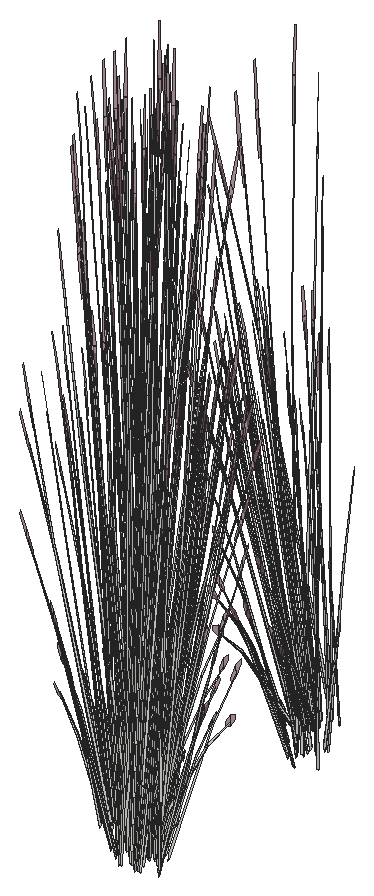
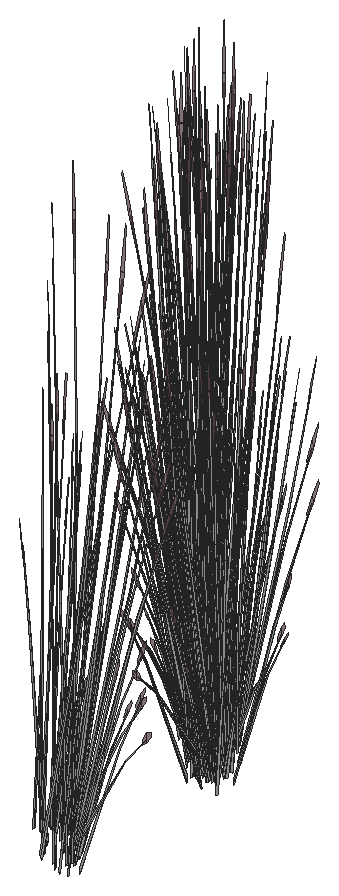
# SketchUp Ruby script. Lengths in inches.
U = 1.inch
M = Sketchup.active_model
def pt(a) = Geom::Point3d.new(a.map { |v| v * U })
def face(e, loops, mat)
  f = e.add_face(loops[0].map { |a| pt(a) })
  loops[1..].each { |l| e.add_face(l.map { |a| pt(a) }).erase! }
  f.material = f.back_material = mat if mat
  f
end
# faces: each face lists its corners as indices into pts; further lists are holes
def faces(e, pts, list, mat = nil) = list.each { |f| face(e, (f[0].is_a?(Array) ? f : [f]).map { |l| l.map { |i| pts[i] } }, mat) }
# xy, xz, yz: faces in a plane at the given z, y or x. An outline is a flat list of corners, or four numbers for a rectangle; further outlines are holes
def ring(l) = l.size == 4 ? [[l[0], l[1]], [l[2], l[1]], [l[2], l[3]], [l[0], l[3]]] : l.each_slice(2).to_a
def flat(e, list, mat, &to3) = list.each { |f| face(e, (f[0].is_a?(Array) ? f : [f]).map { |l| ring(l).map { |u, v| to3.(u, v) } }, mat) }
def xy(e, z, list, mat = nil) = flat(e, list, mat) { |x, y| [x, y, z] }
def xz(e, y, list, mat = nil) = flat(e, list, mat) { |x, z| [x, y, z] }
def yz(e, x, list, mat = nil) = flat(e, list, mat) { |y, z| [x, y, z] }
def lines(e, pts, list) = list.each { |a, b| e.add_line(pt(pts[a]), pt(pts[b])) }
# prism: a flat outline (further loops are holes) pulled along v
def prism(e, loops, v, mat = nil)
  f = face(e, loops, mat); d = Geom::Vector3d.new(v.map { |x| x * U })
  f.pushpull(f.normal.samedirection?(d) ? d.length : -d.length)
end
def box(e, o, s, mat = nil) = prism(e, [[o, [o[0] + s[0], o[1], o[2]], [o[0] + s[0], o[1] + s[1], o[2]], [o[0], o[1] + s[1], o[2]]]], [0, 0, s[2]], mat)
def at(x, y, z, deg = 0) = Geom::Transformation.translation(pt([x, y, z])) * Geom::Transformation.rotation(ORIGIN, Z_AXIS, deg.degrees)
def axes(o, x, y, z) = Geom::Transformation.new([*x, 0, *y, 0, *z, 0, *pt(o).to_a, 1])
def part(name) = M.definitions.add(name)
# library, detail: a bought-in or finely detailed component or shape, given as its bounding box
def library(name, o, s) = part(name).tap { |d| box(d.entities, o, s) }
def detail(e, o, s) = box(e.add_group.entities, o, s)
def put(e, d, t, mat = nil) = e.add_instance(d, t).tap { |i| i.material = mat if mat }
def group(e, t, mat = nil) = e.add_group.tap { |g| g.transformation = t; g.material = mat if mat }.entities
root = M.entities
M.materials.add("LightPink_Translucent").color = [144, 107, 117]
M.materials["LightPink_Translucent"].alpha = 0.75
c1 = part("blade")
p = [[2.15,0.21,22],[0,0.17,0],[0.09,0.45,0],[2.18,0.31,22],[2.29,0.31,22],[0.38,0.45,0],
  [2.48,0.24,33],[2.49,0.24,33],[2.48,0.22,33]]
faces(c1.entities,p,[[0,1,2,3],[4,5,2,3],[6,3,4,7],[8,0,3,6]])
c2 = part("seeds")
p = [[0.3,-0.1,1.38],[-0.01,-0.03,1.59],[-0.01,-0.03,0.03],[0.14,-0.07,-0.07],[0.29,-0.03,3],[0.15,0.01,3.11]]
faces(c2.entities,p,[[0,1,2,3],[1,0,4,5]],"LightPink_Translucent")
c3 = part("blade with seeds")
put(c3.entities,c1,at(0,0,0))
put(c3.entities,c2,axes([2.4,0.25,30.99],[1.5799,-0.05474,1.17369],[-0.12525,1.92788,0.29478],[-0.07173,-0.02425,1.56792]))
put(root,c3,axes([329.61,518.67,1400.59],[0.06891,0.12984,1.43002],[-0.15879,0.35293,-0.30754],[-0.16304,-0.08436,0.61141]))
put(root,c3,axes([330.81,518.05,1400.03],[0.32928,0.11539,-0.30978],[-0.08291,0.40636,0.30978],[0.06638,-0.04686,1.38974]))
put(root,c3,axes([329.89,518.55,1402.98],[-0.35281,-0.01123,-0.71045],[0.0237,-0.47284,0.08574],[-0.14947,-0.0499,1.00501]))
put(root,c3,axes([332.7,519.05,1402.73],[0.2423,0.19613,0.0643],[-0.14107,0.2793,0.50621],[0.07768,-0.0903,0.77189]))
put(root,c3,axes([332.63,518.97,1402.73],[0.08753,0.42921,0.48003],[-0.34336,0.07449,0.3958],[0.1012,-0.10094,0.9933]))
put(root,c3,axes([333.55,519.49,1402.72],[0.04898,-0.07104,1.74944],[-0.06269,-0.43574,-0.27667],[0.12289,-0.08262,0.14031]))
put(root,c3,axes([329.875,519.46,1400.33],[-0.32829,0.39208,0.30756],[-0.32849,-0.38796,-0.36492],[-0.01146,-0.11134,1.64885]))
put(root,c3,axes([329.42,517.78,1402.71],[0.02617,0.04654,1.77383],[-0.12614,0.41836,-0.16761],[-0.12775,0.00303,0.31391]))
put(root,c3,axes([330.92,519.65,1400.43],[0.39767,0.22603,0.24065],[-0.19139,0.46966,0.50002],[0,-0.10827,1.60543]))
put(root,c3,axes([330.77,520.28,1400.4375],[0.09355,-0.55261,-0.23429],[0.44354,0.09633,0.51271],[-0.0775,-0.07631,1.5644]))
put(root,c3,axes([329.78,518.65,1402.68],[-0.25628,0.30892,-0.51099],[-0.22444,-0.32634,-0.3958],[-0.13021,-0.047,0.97773]))
put(root,c3,axes([329.97,518.51,1403.05],[0.20082,0.29199,0.35414],[-0.2293,0.2764,-0.4572],[-0.1165,-0.04206,0.87481]))
put(root,c3,axes([329.2,519.06,1400.77],[0.22533,-0.03337,1.1486],[-0.14293,0.29403,0.84392],[-0.11135,-0.04411,0.25299]))
put(root,c3,axes([330.79,519.33,1400.72],[-0.38326,0.02879,0.44739],[-0.03466,-0.47788,-0.21531],[0.06861,-0.04843,1.43643]))
put(root,c3,axes([329.91,518.33,1403.03],[-0.0189,0.47427,-0.1216],[-0.35781,-0.01296,-0.67495],[-0.13781,-0.03295,1.02557]))
put(root,c3,axes([329.8,519.68,1400.48],[0,0.46636,0.49651],[-0.39487,0,0],[0,-0.10622,1.57504]))
put(root,c3,axes([332.59,520.15,1403.03],[-0.17758,-0.42229,-0.1216],[0.31518,-0.20752,-0.67495],[0.13282,-0.05572,1.02557]))
put(root,c3,axes([332.57,519.78,1402.68],[0.09562,-0.42421,-0.51099],[0.32782,0.1454,-0.3958],[0.13199,-0.0389,0.97773]))
put(root,c3,axes([332.06,518.06,1400.375],[0.22066,-0.46731,0],[0.36918,0.26061,-0.51607],[0.08408,0.05936,1.63711]))
put(root,c3,axes([329.46,518.98,1401.875],[0.14639,-0.01056,1.71376],[-0.09712,0.45778,0.13857],[-0.20862,-0.02831,0.73262]))
put(root,c3,axes([330.73,520.06,1400.21],[-0.21202,-0.39143,-0.44739],[0.32115,-0.27564,0.21531],[-0.06861,-0.04843,1.43643]))
put(root,c3,axes([330.78,519.5,1400.36],[0.15345,0.52148,0.45755],[-0.43845,0.18134,0.17955],[0.00536,-0.09582,1.58856]))
put(root,c3,axes([332.92,519.9,1399.98],[-0.22732,0.05597,1.41583],[-0.03618,-0.44548,0.08104],[0.15921,-0.06743,0.80566]))
put(root,c3,axes([333.34,519.51,1400.26],[-0.21881,-0.29821,-0.06488],[0.23965,-0.27324,-0.29416],[0.0679,-0.01924,0.97024]))
put(root,c3,axes([330.7,519.91,1400.72],[-0.17124,0.42022,0.44739],[-0.35581,-0.20224,-0.21531],[0,-0.09687,1.43643]))
put(root,c3,axes([331.33,519.55,1400.21],[0,-0.53961,0],[0.44133,0,0],[0,0,1.79456]))
put(root,c3,axes([331.87,518.3,1400.48],[-0.33032,-0.23318,0.49651],[0.19744,-0.41812,0],[0.07523,0.05311,1.57504]))
put(root,c3,axes([332.51,519.9375,1402.98],[0.31014,-0.20596,-0.71045],[0.17284,0.42397,0.08574],[0.14985,-0.04816,1.00501]))
put(root,c3,axes([330.54,520.21,1400.06],[-0.36714,-0.07646,-0.62353],[0.07747,-0.47163,-0.16365],[-0.10956,-0.05715,1.37633]))
put(root,c3,axes([331.12,519.21,1400.36],[-0.29264,0.42323,0.45755],[-0.34767,-0.3736,0.17955],[0.07055,-0.04224,1.58856]))
put(root,c3,axes([331.44,519.97,1400.3],[-0.32829,-0.4014,-0.06131],[0.32849,-0.40164,0],[-0.01146,-0.01402,1.75571]))
put(root,c3,axes([330.61,518.51,1400.47],[-0.10196,0.46348,0.17642],[-0.3731,-0.13116,0.35086],[0.06445,-0.00226,1.60407]))
put(root,c3,axes([332.47,520.02,1403.05],[-0.29332,-0.1301,0.35414],[0.08555,-0.37955,-0.4572],[0.11809,-0.0348,0.87481]))
put(root,c3,axes([329.4,519.33,1402.73],[0.09971,-0.42522,0.48003],[0.32782,0.1454,0.3958],[-0.12892,0.02555,0.9933]))
put(root,c3,axes([330.46,518.89,1399.59],[-0.3474,0.18671,1.28929],[-0.11057,-0.53572,0.50096],[0.21332,0.00891,1.46642]))
put(root,c3,axes([331.39,519.03,1400.62],[0.06809,-0.4162,0.1448],[0.33266,0.07225,-0.41347],[0.06054,0.04274,1.26744]))
put(root,c3,axes([329.37,519.21,1402.73],[-0.12963,-0.31798,0.0643],[0.23638,-0.15564,0.50621],[-0.1042,0.03071,0.77189]))
put(root,c3,axes([330.82,520.02,1400.36],[0.44609,0.09826,0.45755],[-0.09078,0.55493,0.17955],[-0.06519,-0.05359,1.58856]))
put(root,c3,axes([333.17,519.61,1399.49],[-0.01845,-0.0708,1.76342],[0.12793,-0.41416,-0.26939],[0.12905,-0.00596,0.30037]))
put(root,c3,axes([329.36,519.54,1399.49],[0.00895,0.0735,1.76342],[-0.18044,0.38382,-0.26939],[-0.12817,-0.01935,0.30037]))
put(root,c3,axes([331.25,519.14,1400.72],[-0.21202,-0.39143,0.44739],[0.32115,-0.27564,-0.21531],[0.06861,0.04843,1.43643]))
put(root,c3,axes([330.15,520.93,1400.03],[-0.08291,-0.40636,-0.30978],[0.32928,-0.11539,0.30978],[-0.06638,-0.04686,1.38974]))
put(root,c3,axes([330.58,520.9,1400.47],[0.37926,-0.12378,0.17642],[0.09365,0.46065,0.35086],[-0.03382,-0.06712,1.60407]))
put(root,c3,axes([331.36,519.16,1400.67],[0.35635,-0.30962,-0.29095],[0.23697,0.43749,-0.50002],[0.08792,0.04443,1.59708]))
put(root,c3,axes([332.78,519.98,1402.53],[0.29332,0.1301,-0.35414],[-0.08555,0.37955,0.4572],[0.11809,-0.0348,0.87481]))
put(root,c3,axes([330.0625,521.1,1400.02],[-0.33032,-0.23318,-0.49651],[0.19744,-0.41812,0],[-0.07523,-0.05311,1.57504]))
put(root,c3,axes([332.26,518.34,1400.02],[0.33032,0.23318,-0.49651],[-0.19744,0.41812,0],[0.07523,0.05311,1.57504]))
put(root,c3,axes([329.33,519.375,1402.53],[-0.29332,-0.1301,-0.35414],[0.08555,-0.37955,0.4572],[-0.11809,0.0348,0.87481]))
put(root,c3,axes([331.63,519.67,1400.21],[0.39487,0,0],[0,0.48281,0],[0,0,1.78407]))
put(root,c3,axes([330.96,520.28,1400.67],[-0.35635,0.30962,-0.29095],[-0.23697,-0.43749,-0.50002],[-0.08792,-0.04443,1.59708]))
put(root,c3,axes([331.74,518.54,1400.47],[-0.37926,0.12378,0.17642],[-0.09365,-0.46065,0.35086],[0.03382,0.06712,1.60407]))
put(root,c3,axes([331.98,519.51,1401.875],[-0.14639,0.01056,1.71376],[0.09712,-0.45778,0.13857],[0.20862,0.02831,0.73262]))
put(root,c3,axes([332.17,518.51,1400.03],[0.08291,0.40636,-0.30978],[-0.32928,0.11539,0.30978],[0.06638,0.04686,1.38974]))
put(root,c3,axes([332.73,520.14,1402.73],[0.12963,0.31798,0.0643],[-0.23638,0.15564,0.50621],[0.1042,-0.03071,0.77189]))
put(root,c3,axes([331.5,519.42,1400.38],[-0.44609,-0.09826,0.49198],[0.09078,-0.55493,0.19306],[0.06519,0.05359,1.70813]))
put(root,c3,axes([332.71,520.02,1402.73],[-0.09971,0.42522,0.48003],[-0.32782,-0.1454,0.3958],[0.12892,-0.02555,0.9933]))
put(root,c3,axes([331.15,520.79,1400.2],[-0.11516,-0.40207,0],[0.32884,-0.1408,0],[0,0,1.54371]))
put(root,c3,axes([330.93,520.41,1400.62],[-0.06809,0.4162,0.1448],[-0.33266,-0.07225,-0.41347],[-0.06054,-0.04274,1.26744]))
put(root,c3,axes([329.64,519.33,1403.05],[0.29332,0.1301,0.35414],[-0.08555,0.37955,-0.4572],[-0.11809,0.0348,0.87481]))
put(root,c3,axes([331.58,520.74,1400.18],[0.37054,-0.15823,-0.19198],[0.1302,0.45581,0.00008],[0.0409,-0.01749,1.73897]))
put(root,c3,axes([331.71,520.93,1400.47],[0.10196,-0.46348,0.17642],[0.3731,0.13116,0.35086],[-0.06445,0.00226,1.60407]))
put(root,c3,axes([331.62,519.875,1400.21],[0.24637,0.30123,0],[-0.24637,0.30123,0],[0,0,1.69266]))
put(root,c3,axes([330.22,519.31,1401.34],[0.10032,-0.06746,1.77064],[0.0346,0.47103,0.13857],[-0.2173,0.0625,0.63284]))
put(root,c3,axes([332.29,519.74,1400.47],[-0.2773,-0.3397,0.17642],[0.27945,-0.32949,0.35086],[-0.03063,0.06937,1.60407]))
put(root,c3,axes([331.78,519.23,1400.06],[0.36714,0.07646,-0.62353],[-0.07747,0.47163,-0.16365],[0.10956,0.05715,1.37633]))
put(root,c3,axes([333.4,520.06,1400.77],[-0.21807,0.07699,1.1486],[0.10265,-0.31819,0.84392],[0.11568,0.02177,0.25299]))
put(root,c3,axes([331.07,520.97,1400.2],[-0.35581,-0.20937,0],[0.17124,-0.43505,0],[0,0,1.62707]))
put(root,c3,axes([331.36,520.42,1400.46],[-0.34464,-0.37536,-0.25192],[0.29,-0.42149,0.5513],[-0.0928,0.04391,1.68216]))
put(root,c3,axes([330.45,521.14,1400.48],[0.33032,0.23318,0.49651],[-0.19744,0.41812,0],[-0.07523,-0.05311,1.57504]))
put(root,c3,axes([331.62,519.52,1400.72],[0.17124,-0.42022,0.44739],[0.35581,0.20224,-0.21531],[0,0.09687,1.43643]))
put(root,c3,axes([333.3,521.4,1402.71],[-0.03191,-0.04083,1.77383],[0.06981,-0.43764,-0.16761],[0.12571,-0.02796,0.31391]))
put(root,c3,axes([329.14,519.625,1402.72],[-0.05763,0.06055,1.74944],[0.0049,0.44239,-0.27667],[-0.13211,0.05753,0.14031]))
put(root,c3,axes([331.55,519.76,1400.29],[0,0.53934,-0.05637],[-0.44133,0,0],[0,0.01695,1.79368]))
put(root,c3,axes([329.53,519.57,1402.68],[-0.09562,0.42421,-0.51099],[-0.32782,-0.1454,-0.3958],[-0.13199,0.0389,0.97773]))
put(root,c3,axes([329.51,519.2,1403.03],[0.17758,0.42229,-0.1216],[-0.31518,0.20752,-0.67495],[-0.13282,0.05572,1.02557]))
put(root,c3,axes([331.58,519.38,1400.21],[0.21202,0.39143,-0.44739],[-0.32115,0.27564,0.21531],[0.06861,0.04843,1.43643]))
put(root,c3,axes([333.02,521.04,1401.93],[-0.06755,-0.39203,-0.03492],[0.31928,-0.09013,-0.15832],[0.06667,0.02485,0.52218]))
put(root,c3,axes([330.26,521.38,1400.375],[-0.22066,0.46731,0],[-0.36918,-0.26061,-0.51607],[-0.08408,-0.05936,1.63711]))
put(root,c3,axes([332.19,521.02,1403.03],[0.0189,-0.47427,-0.1216],[0.35781,0.01296,-0.67495],[0.13781,0.03295,1.02557]))
put(root,c3,axes([332.52,519.76,1400.48],[0,-0.46636,0.49651],[0.39487,0,0],[0,0.10622,1.57504]))
put(root,c3,axes([331.53,520.11,1400.72],[0.38326,-0.02879,0.44739],[0.03466,0.47788,-0.21531],[-0.06861,0.04843,1.43643]))
put(root,c3,axes([331.77,519.62,1400.62],[0.32884,-0.136,0.1448],[0.11516,0.38837,-0.41347],[0,0.08547,1.26744]))
put(root,c3,axes([332.14,520.84,1403.05],[-0.20082,-0.29199,0.35414],[0.2293,-0.2764,-0.4572],[0.1165,0.04206,0.87481]))
put(root,c3,axes([331.1875,520.34,1400.21],[-0.38326,0.02879,-0.44739],[-0.03466,-0.47788,0.21531],[-0.06861,0.04843,1.43643]))
put(root,c3,axes([332.99,520.57,1400.59],[-0.085,-0.1147,1.43002],[0.1106,-0.37943,-0.30754],[0.17198,0.0514,0.61141]))
put(root,c3,axes([331.47,520.98,1400.2],[0.35581,0.20937,0],[-0.17124,0.43505,0],[0,0,1.74954]))
put(root,c3,axes([332.5,520.74,1402.72],[0.07571,-0.00789,1.74944],[0.20767,-0.36231,-0.27667],[0.13467,0.04783,0.14031]))
put(root,c3,axes([331.61,521.45,1400.19],[-0.21791,-0.46895,-0.05142],[0.36918,-0.26061,0.51607],[-0.09097,0.04465,1.6363]))
put(root,c3,axes([331.53,520.3125,1400.62],[0.26075,0.2802,0.1448],[-0.2175,0.31612,-0.41347],[-0.06054,0.04274,1.26744]))
put(root,c3,axes([329.47,520.39,1402.73],[-0.08753,-0.42921,0.48003],[0.34336,-0.07449,0.3958],[-0.1012,0.10094,0.9933]))
put(root,c3,axes([329.41,520.3,1402.73],[-0.2423,-0.19613,0.0643],[0.14107,-0.2793,0.50621],[-0.07768,0.0903,0.77189]))
put(root,c3,axes([329.52,519.79,1401.875],[0.12246,-0.09864,1.71376],[0.1031,0.45582,0.13857],[-0.19225,0.10302,0.73262]))
put(root,c3,axes([332.21,520.8,1402.98],[0.35281,0.01123,-0.71045],[-0.0237,0.47284,0.08574],[0.14947,0.0499,1.00501]))
put(root,c3,axes([331.8125,521.18,1400.48],[0.33032,-0.23318,0.49651],[0.19744,0.41812,0],[-0.07523,0.05311,1.57504]))
put(root,c3,axes([331.34,520.81,1400.29],[0.15345,0.53576,-0.06012],[-0.43845,0.18773,0],[0.00536,0.01871,1.72173]))
put(root,c3,axes([331.51,521.39,1400.03],[-0.32928,-0.11539,-0.30978],[0.08291,-0.40636,0.30978],[-0.06638,0.04686,1.38974]))
put(root,c3,axes([329.14,520.5625,1400.59],[0.12266,0.03828,1.43002],[0.07906,0.39104,-0.30754],[-0.16661,0.0732,0.61141]))
put(root,c3,axes([329.6875,520.24,1403.05],[0.30722,-0.06665,0.35414],[0.08112,0.381,-0.4572],[-0.08804,0.10234,0.87481]))
put(root,c3,axes([332.78,519.84,1400.375],[0.44133,0,0],[0,0.52122,-0.51607],[0,0.11871,1.63711]))
put(root,c3,axes([328.5,520.07,1402.71],[0.04504,0.01251,1.77383],[0.13934,0.41205,-0.16761],[-0.0922,0.10815,0.31391]))
put(root,c3,axes([332.61,520.1,1400.2],[-0.44111,-0.00373,-0.04976],[0,-0.52122,0.49943],[-0.01386,0.11865,1.58352]))
put(root,c3,axes([331.65,519.65,1400.67],[0.39748,0.22252,-0.29095],[-0.19139,0.46966,-0.50002],[0.01249,0.11531,1.59708]))
put(root,c3,axes([328.88,521.38,1400.77],[0.14709,-0.21136,1.1486],[0.05804,0.3346,0.84392],[-0.1063,0.05991,0.25299]))
put(root,c3,axes([332.42,520.99,1402.53],[0.20082,0.29199,-0.35414],[-0.2293,0.2764,0.4572],[0.1165,0.04206,0.87481]))
put(root,c3,axes([332.52,520.18,1400.03],[-0.24637,0.29097,-0.30978],[-0.24637,-0.29097,0.30978],[0,0.09372,1.38974]))
put(root,c3,axes([331.46,520.21,1400.67],[0.04113,0.53214,-0.29095],[-0.42835,0.03218,-0.50002],[-0.07543,0.07088,1.59708]))
put(root,c3,axes([332.32,521.1,1402.73],[-0.01777,0.35463,0.0643],[-0.26836,-0.00972,0.50621],[0.1028,0.03711,0.77189]))
put(root,c3,axes([331.61,520,1400.21],[-0.17124,0.42022,-0.44739],[-0.35581,-0.20224,0.21531],[0,0.09687,1.43643]))
put(root,c3,axes([329.43,520.47,1402.53],[-0.30722,0.06665,-0.35414],[-0.08112,-0.381,0.4572],[-0.08804,0.10234,0.87481]))
put(root,c3,axes([332.34,520.99,1402.73],[-0.26024,0.30729,0.48003],[-0.22444,-0.32634,0.3958],[0.1221,0.05668,0.9933]))
put(root,c3,axes([328.99,521.32,1403.65],[0.31145,0.12449,-0.06488],[-0.0958,0.38314,-0.29416],[-0.05094,0.05817,0.97024]))
put(root,c3,axes([331.2,520.61,1400.06],[-0.23773,0.35053,-0.62353],[-0.29532,-0.31785,-0.16365],[-0.09526,0.08744,1.37633]))
put(root,c3,axes([331.52,521.35,1403.05],[-0.05451,-0.37564,0.35414],[0.31161,-0.09919,-0.4572],[0.0837,0.10765,0.87481]))
put(root,c3,axes([331.62,521.21,1400.33],[0.44186,0.15158,0.30756],[-0.11054,0.54181,-0.36492],[-0.07313,0.06781,1.64885]))
put(root,c3,axes([331.59,521.57,1400.02],[-0.33032,0.23318,-0.49651],[-0.19744,-0.41812,0],[-0.07523,0.05311,1.57504]))
put(root,c3,axes([332.6875,520.19,1400.02],[0,0.46636,-0.49651],[-0.39487,0,0],[0,0.10622,1.57504]))
put(root,c3,axes([331.7,520.24,1401.875],[-0.1311,-0.08035,1.71376],[0.27131,-0.33708,0.13857],[0.16909,0.15206,0.73262]))
put(root,c3,axes([331.72,519.18,1402.47],[-0.30498,-0.24231,1.38283],[0.32203,-0.37727,0.59665],[0.0984,0.22736,1.33663]))
put(root,c3,axes([329.53,520.21,1403.03],[0.32648,0.25715,-0.1216],[-0.18809,0.3724,-0.67495],[-0.09224,0.12945,1.02557]))
put(root,c3,axes([332.18,521.16,1400.77],[-0.19872,-0.13409,1.1486],[0.2566,-0.13625,0.84392],[0.06921,0.11541,0.25299]))
put(root,c3,axes([331.49,521.54,1403.03],[0.21031,-0.39918,-0.1216],[0.30457,0.22997,-0.67495],[0.10587,0.11278,1.02557]))
put(root,c3,axes([329.97,520.09,1401.875],[0.08815,-0.14329,1.71376],[0.22258,0.38678,0.13857],[-0.15267,0.17614,0.73262]))
put(root,c3,axes([329.6875,520.51,1402.68],[0.09067,0.42583,-0.51099],[-0.34336,0.07449,-0.3958],[-0.0984,0.11438,0.97773]))
put(root,c3,axes([330.1,521,1403.05],[0.23881,-0.24554,0.35414],[0.22606,0.28036,-0.4572],[-0.0344,0.14245,0.87481]))
put(root,c3,axes([331.89,521.5,1400.375],[0.22066,0.46731,0],[-0.36918,0.26061,-0.51607],[-0.08408,0.05936,1.63711]))
put(root,c3,axes([331.21,521.87,1402.71],[0.00104,-0.05646,1.77383],[0.30246,-0.2491,-0.16761],[0.10506,0.08891,0.31391]))
put(root,c3,axes([332.24,521.66,1399.49],[0.02571,-0.06733,1.76342],[0.32373,-0.19829,-0.26939],[0.09815,0.10263,0.30037]))
put(root,c3,axes([331.7,519.65,1400.84],[-0.00964,-0.43909,1.41272],[0.43635,0.11382,0.59816],[-0.1032,0.24027,1.3335]))
put(root,c3,axes([331.8125,520.125,1400.09],[0.12941,0.42699,-0.69212],[-0.37279,0.15378,-0.18165],[0.0143,0.14459,1.52773]))
put(root,c3,axes([329.88,521.22,1402.73],[-0.29004,-0.02173,0.0643],[0.00795,-0.32812,0.50621],[-0.03035,0.12569,0.77189]))
put(root,c3,axes([329.27,521.6,1399.49],[0.04734,0.04659,1.76342],[0.08027,0.4317,-0.26939],[-0.10492,0.09206,0.30037]))
put(root,c3,axes([329.98,521.25,1402.73],[-0.25132,-0.3182,0.48003],[0.2669,-0.27442,0.3958],[-0.04636,0.14929,0.9933]))
put(root,c3,axes([331.74,521.34,1402.68],[0.34827,-0.11086,-0.51099],[0.06092,0.41983,-0.3958],[0.09354,0.12031,0.97773]))
put(root,c3,axes([330.77,521.41,1403.05],[0.1064,-0.35863,0.35414],[0.31043,0.1046,-0.4572],[0.02846,0.14439,0.87481]))
put(root,c3,axes([332.22,521.77,1400.67],[-0.22633,-0.01463,1.0506],[0.14947,-0.31064,0.58006],[0.08941,0.11036,0.8241]))
put(root,c3,axes([331.56,521.6875,1402.73],[-0.16041,0.29625,0.0643],[-0.22843,-0.17248,0.50621],[0.07385,0.09498,0.77189]))
put(root,c3,axes([331.1875,522.68,1403.65],[0.2439,-0.26754,-0.06488],[0.22348,0.29302,-0.29416],[0.01573,0.08303,0.97024]))
put(root,c3,axes([331.63,521.6,1402.73],[-0.35104,0.10702,0.48003],[-0.06092,-0.41983,0.3958],[0.08256,0.12373,0.9933]))
put(root,c3,axes([329.9,520.45,1401.875],[0.06572,-0.16029,1.71376],[0.27569,0.33172,0.13857],[-0.12437,0.20675,0.73262]))
put(root,c3,axes([331.48,521.01,1400.59],[0.00623,-0.15459,1.43002],[0.29764,-0.17268,-0.30754],[0.09188,0.18503,0.61141]))
put(root,c3,axes([330.67,521.73,1402.73],[-0.26007,0.1585,0.0643],[-0.12729,-0.28902,0.50621],[0.02512,0.1274,0.77189]))
put(root,c3,axes([329.98,521.35,1402.53],[-0.23881,0.24554,-0.35414],[-0.22606,-0.28036,0.4572],[-0.0344,0.14245,0.87481]))
put(root,c3,axes([329.15,521.28,1402.72],[-0.00877,0.09229,1.74944],[0.24897,0.32105,-0.27667],[-0.06518,0.15182,0.14031]))
put(root,c3,axes([329.95,521.07,1403.4],[0.3879,0.02311,-0.13498],[-0.0106,0.43749,-0.74919],[-0.02694,0.1685,1.13838]))
put(root,c3,axes([330.67,521.56,1403.03],[0.34538,-0.21713,-0.1216],[0.16972,0.38536,-0.67495],[0.04557,0.16239,1.02557]))
put(root,c3,axes([330.77,521.7,1403.0625],[-0.34777,-0.12192,0.53283],[0.11892,-0.40083,0.43934],[0.0209,0.15763,1.10256]))
put(root,c3,axes([330.13,522.3,1400.77],[-0.00913,-0.2773,1.1486],[0.22824,0.19778,0.84392],[-0.04489,0.13217,0.25299]))
put(root,c3,axes([330.73,521.64,1399.49],[0.05712,-0.02538,1.76342],[0.34359,0.13968,-0.26939],[0.01005,0.15742,0.30037]))
put(root,c3,axes([330.21,521.23,1403],[0.25266,0.31335,-0.5672],[-0.2669,0.27442,-0.43934],[-0.03844,0.15921,1.08528]))
put(root,c3,axes([329.9375,521.7,1400.82],[0.32063,-0.08258,0.06507],[0.07371,0.33271,-0.86304],[-0.02033,0.16842,0.7736]))
put(root,c3,axes([330.96,521.54,1402.68],[0.34695,0.11691,-0.51099],[-0.11892,0.40083,-0.3958],[0.03181,0.16138,0.97773]))
put(root,c3,axes([331.16,520.71,1401.875],[-0.08068,-0.14973,1.71376],[0.3728,-0.12606,0.13857],[0.08426,0.23506,0.73262]))
put(root,c3,axes([330.8,521.78,1402.53],[-0.1064,0.35863,-0.35414],[-0.31043,-0.1046,0.4572],[0.02846,0.14439,0.87481]))
put(root,c3,axes([330.13,521.09,1403.34],[-0.00918,0.43138,-0.7886],[-0.38672,-0.02897,0.09517],[-0.04081,0.18275,1.11556]))
put(root,c3,axes([329.125,522.22,1402.71],[0.04004,-0.02816,1.77383],[0.33095,0.18728,-0.16761],[-0.00778,0.15594,0.31391]))
put(root,c3,axes([330.5,520.78,1401.875],[-0.00864,-0.17899,1.71376],[0.37441,0.11874,0.13857],[-0.02316,0.25508,0.73262]))
put(root,c3,axes([330.84,521.46,1402.98],[0.16845,0.3792,-0.71045],[-0.34676,0.21133,0.08574],[0.03939,0.18322,1.00501]))
put(root,c3,axes([329.86,522.06,1400.59],[0.11138,-0.07357,1.43002],[0.27499,0.22183,-0.30754],[-0.08185,0.19194,0.61141]))
put(root,c3,axes([330.58,522.42,1402.72],[0.04474,0.0751,1.74944],[0.36104,0.0295,-0.27667],[0.03631,0.16562,0.14031]))
put(root,c3,axes([330.01,521.7,1401.36],[0.00775,-0.24075,1.54345],[0.34877,0.12716,0.21329],[-0.03022,0.25658,0.72882]))
put(root,c3,axes([330.27,537.89,1401.875],[0.08068,0.14973,1.71376],[-0.3728,0.12606,0.13857],[-0.08426,-0.23506,0.73262]))
put(root,c3,axes([330.89,536.9,1402.72],[-0.05398,-0.06539,1.74944],[-0.36026,0.04145,-0.27667],[-0.0575,-0.15639,0.14031]))
put(root,c3,axes([331.72,537.67,1400.59],[-0.10032,0.0944,1.43002],[-0.30046,-0.16522,-0.30754],[0.05569,-0.20547,0.61141]))
put(root,c3,axes([331.27,538,1402.98],[-0.16845,-0.3792,-0.71045],[0.34676,-0.21133,0.08574],[-0.03939,-0.18322,1.00501]))
put(root,c3,axes([330.17,537.49,1400.59],[-0.02137,0.15256,1.43002],[-0.31245,0.12771,-0.30754],[-0.07303,-0.19719,0.61141]))
put(root,c3,axes([330.98,537.16,1399.49],[-0.0592,0.0168,1.76342],[-0.32738,-0.18913,-0.26939],[0.00549,-0.15776,0.30037]))
put(root,c3,axes([331.97,538.37,1402.98],[0.00918,-0.43138,-0.71045],[0.38672,0.02897,0.08574],[0.04081,-0.18275,1.00501]))
put(root,c3,axes([332.51,537.7,1402.72],[-0.00341,-0.09282,1.74944],[-0.28775,-0.26825,-0.27667],[0.04449,-0.16261,0.14031]))
put(root,c3,axes([331.3,537.68,1402.53],[0.1064,-0.35863,-0.35414],[0.31043,0.1046,0.4572],[-0.02846,-0.14439,0.87481]))
put(root,c3,axes([331.53,538.15,1401.875],[-0.06572,0.16029,1.71376],[-0.27569,-0.33172,0.13857],[0.12437,-0.20675,0.73262]))
put(root,c3,axes([332.43,537.37,1402.71],[-0.03584,0.03562,1.77383],[-0.35118,-0.12018,-0.16761],[-0.01271,-0.15545,0.31391]))
put(root,c3,axes([331.14,537.93,1402.68],[-0.34695,-0.11691,-0.51099],[0.11892,-0.40083,-0.3958],[-0.03181,-0.16138,0.97773]))
put(root,c3,axes([331.35,536.92,1400.77],[0.04528,0.27194,1.1486],[-0.25117,-0.15062,0.84392],[0.02703,-0.13924,0.25299]))
put(root,c3,axes([331.89,538.23,1402.68],[-0.25266,-0.31335,-0.51099],[0.2669,-0.27442,-0.3958],[0.03844,-0.15921,0.97773]))
put(root,c3,axes([330.52,536.68,1402.71],[-0.00658,0.0559,1.77383],[-0.32474,0.20287,-0.16761],[-0.09556,-0.1037,0.31391]))
put(root,c3,axes([330.45,537.68,1403.09],[0.39316,-0.11987,0.53763],[0.06823,0.47021,0.4433],[-0.09247,-0.13858,1.11249]))
put(root,c3,axes([331.34,537.76,1402.73],[0.34777,0.12192,0.48003],[-0.11892,0.40083,0.3958],[-0.0209,-0.15763,0.9933]))
put(root,c3,axes([331.4375,537.91,1403.03],[-0.34538,0.21713,-0.1216],[-0.16972,-0.38536,-0.67495],[-0.04557,-0.16239,1.02557]))
put(root,c3,axes([332.15,538.39,1403.03],[-0.3879,-0.02311,-0.1216],[0.0106,-0.43749,-0.67495],[0.02694,-0.1685,1.02557]))
put(root,c3,axes([332.13,538.11,1402.53],[0.23881,-0.24554,-0.35414],[0.22606,0.28036,0.4572],[0.0344,-0.14245,0.87481]))
put(root,c3,axes([330.0625,537.25,1400.77],[0.18411,0.16231,1.1486],[-0.26813,0.09757,0.84392],[-0.05737,-0.12474,0.25299]))
put(root,c3,axes([331.43,537.73,1402.73],[0.26007,-0.1585,0.0643],[0.12729,0.28902,0.50621],[-0.02512,-0.1274,0.77189]))
put(root,c3,axes([330.51,538.11,1402.98],[-0.30095,-0.22541,-0.71045],[0.21388,-0.395,0.08574],[-0.10904,-0.13459,1.00501]))
put(root,c3,axes([330.4,537.8125,1402.53],[-0.05451,-0.37564,-0.35414],[0.31161,-0.09919,0.4572],[-0.0837,-0.10765,0.87481]))
put(root,c3,axes([330.54,537.78,1402.73],[0.16041,-0.29625,0.0643],[0.22843,0.17248,0.50621],[-0.07385,-0.09498,0.77189]))
put(root,c3,axes([329.92,537.74,1399.49],[-0.03419,0.06144,1.76342],[-0.3455,0.13246,-0.26939],[-0.08346,-0.12049,0.30037]))
put(root,c3,axes([330.49,539.43,1400.1],[-0.14494,-0.47823,-0.69835],[0.41752,-0.17223,-0.18329],[-0.01602,-0.16194,1.54149]))
put(root,c3,axes([329.73,538.36,1401.875],[0.1311,0.08035,1.71376],[-0.27131,0.33708,0.13857],[-0.16909,-0.15206,0.73262]))
put(root,c3,axes([332.43,537.96,1399.49],[-0.05283,-0.03674,1.76342],[-0.13569,-0.41045,-0.26939],[0.09154,-0.11138,0.30037]))
put(root,c3,axes([331.33,538.06,1403.05],[-0.1064,0.35863,0.35414],[-0.31043,-0.1046,-0.4572],[-0.02846,-0.14439,0.87481]))
put(root,c3,axes([330.37,538.12,1402.68],[-0.34827,0.11086,-0.51099],[-0.06092,-0.41983,-0.3958],[-0.09354,-0.12031,0.97773]))
put(root,c3,axes([332.125,538.21,1402.73],[0.25132,0.3182,0.48003],[-0.2669,0.27442,0.3958],[0.04636,-0.14929,0.9933]))
put(root,c3,axes([330.61,537.75,1403.43],[-0.23555,0.44708,-0.13619],[-0.34112,-0.25757,-0.75594],[-0.11858,-0.12631,1.14864]))
put(root,c3,axes([332.22,538.24,1402.73],[0.29004,0.02173,0.0643],[-0.00795,0.32812,0.50621],[0.03035,-0.12569,0.77189]))
put(root,c3,axes([332,538.46,1403.05],[-0.23881,0.24554,0.35414],[-0.22606,-0.28036,-0.4572],[0.0344,-0.14245,0.87481]))
put(root,c3,axes([332.42,539.12,1402.98],[0.18436,-0.36797,-0.71045],[0.32306,0.26151,0.08574],[0.11008,-0.13332,1.00501]))
put(root,c3,axes([330.43,538.05,1400.375],[-0.22066,-0.46731,0],[0.36918,-0.26061,-0.51607],[0.08408,-0.05936,1.63711]))
put(root,c3,axes([332.41,538.95,1402.68],[-0.09067,-0.42583,-0.51099],[0.34336,-0.07449,-0.3958],[0.0984,-0.11438,0.97773]))
put(root,c3,axes([330.92,537.49,1400.13],[-0.2439,0.26754,-0.03893],[-0.22348,-0.29302,-0.17649],[-0.01573,-0.08303,0.58215]))
put(root,c3,axes([329.71,537.62,1402.72],[-0.07594,-0.00329,1.74944],[-0.24177,0.32918,-0.27667],[-0.129,-0.06726,0.14031]))
put(root,c3,axes([332.58,539.26,1403.03],[-0.32648,-0.25715,-0.1216],[0.18809,-0.3724,-0.67495],[0.09224,-0.12945,1.02557]))
put(root,c3,axes([331.23,540.66,1401.33],[0.305,0.18805,1.51261],[-0.29879,0.40513,0.59816],[-0.13384,-0.24012,1.26806]))
put(root,c3,axes([330.59,538.12,1403.05],[0.05451,0.37564,0.35414],[-0.31161,0.09919,-0.4572],[-0.0837,-0.10765,0.87481]))
put(root,c3,axes([329.63,539.36,1400.02],[0,-0.46636,-0.49651],[0.39487,0,0],[0,-0.10622,1.57504]))
put(root,c3,axes([330.73,537.98,1400.02],[0.33032,-0.23318,-0.49651],[0.19744,0.41812,0],[0.07523,-0.05311,1.57504]))
put(root,c3,axes([332.69,538.78,1400.59],[-0.12609,-0.01381,1.43002],[-0.12917,-0.37055,-0.30754],[0.1549,-0.10482,0.61141]))
put(root,c3,axes([329.65,538.36,1403.09],[0.29147,-0.34417,0.53763],[0.25138,0.3655,0.4433],[-0.13675,-0.06349,1.11249]))
put(root,c3,axes([333.38,539.14,1402.71],[-0.0461,-0.00354,1.77383],[-0.19143,-0.37951,-0.16761],[0.07688,-0.12478,0.31391]))
put(root,c3,axes([331.12,538.94,1400.06],[0.23773,-0.35053,-0.62353],[0.29532,0.31785,-0.16365],[0.09526,-0.08744,1.37633]))
put(root,c3,axes([332.84,538.1,1400.77],[-0.11756,0.2374,1.1486],[-0.10105,-0.31895,0.84392],[0.09709,-0.07992,0.25299]))
